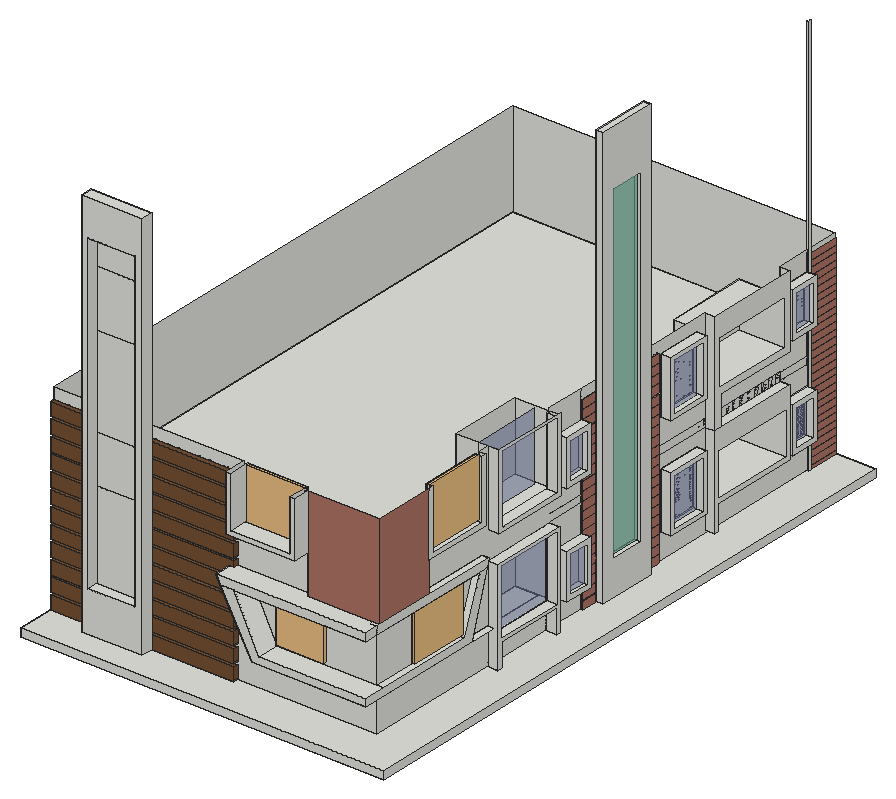
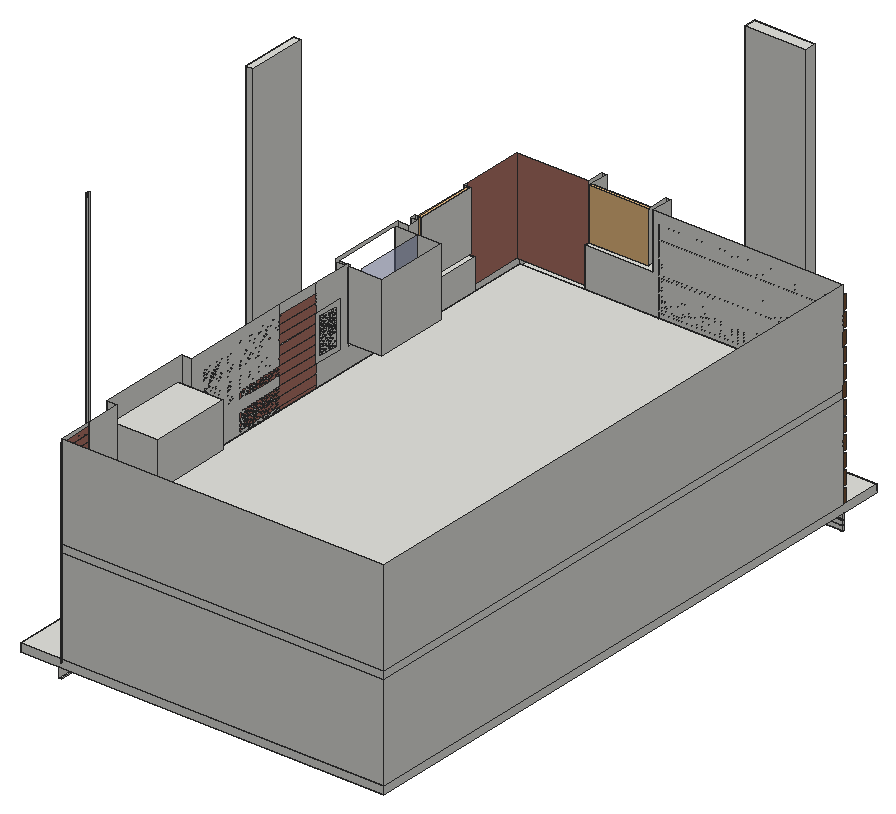
# SketchUp Ruby script. Lengths in inches.
U = 1.inch
M = Sketchup.active_model
def pt(a) = Geom::Point3d.new(a.map { |v| v * U })
def face(e, loops, mat)
  f = e.add_face(loops[0].map { |a| pt(a) })
  loops[1..].each { |l| e.add_face(l.map { |a| pt(a) }).erase! }
  f.material = f.back_material = mat if mat
  f
end
# faces: each face lists its corners as indices into pts; further lists are holes
def faces(e, pts, list, mat = nil) = list.each { |f| face(e, (f[0].is_a?(Array) ? f : [f]).map { |l| l.map { |i| pts[i] } }, mat) }
# xy, xz, yz: faces in a plane at the given z, y or x. An outline is a flat list of corners, or four numbers for a rectangle; further outlines are holes
def ring(l) = l.size == 4 ? [[l[0], l[1]], [l[2], l[1]], [l[2], l[3]], [l[0], l[3]]] : l.each_slice(2).to_a
def flat(e, list, mat, &to3) = list.each { |f| face(e, (f[0].is_a?(Array) ? f : [f]).map { |l| ring(l).map { |u, v| to3.(u, v) } }, mat) }
def xy(e, z, list, mat = nil) = flat(e, list, mat) { |x, y| [x, y, z] }
def xz(e, y, list, mat = nil) = flat(e, list, mat) { |x, z| [x, y, z] }
def yz(e, x, list, mat = nil) = flat(e, list, mat) { |y, z| [x, y, z] }
def lines(e, pts, list) = list.each { |a, b| e.add_line(pt(pts[a]), pt(pts[b])) }
# prism: a flat outline (further loops are holes) pulled along v
def prism(e, loops, v, mat = nil)
  f = face(e, loops, mat); d = Geom::Vector3d.new(v.map { |x| x * U })
  f.pushpull(f.normal.samedirection?(d) ? d.length : -d.length)
end
def box(e, o, s, mat = nil) = prism(e, [[o, [o[0] + s[0], o[1], o[2]], [o[0] + s[0], o[1] + s[1], o[2]], [o[0], o[1] + s[1], o[2]]]], [0, 0, s[2]], mat)
def at(x, y, z, deg = 0) = Geom::Transformation.translation(pt([x, y, z])) * Geom::Transformation.rotation(ORIGIN, Z_AXIS, deg.degrees)
def axes(o, x, y, z) = Geom::Transformation.new([*x, 0, *y, 0, *z, 0, *pt(o).to_a, 1])
def part(name) = M.definitions.add(name)
# library, detail: a bought-in or finely detailed component or shape, given as its bounding box
def library(name, o, s) = part(name).tap { |d| box(d.entities, o, s) }
def detail(e, o, s) = box(e.add_group.entities, o, s)
def put(e, d, t, mat = nil) = e.add_instance(d, t).tap { |i| i.material = mat if mat }
def group(e, t, mat = nil) = e.add_group.tap { |g| g.transformation = t; g.material = mat if mat }.entities
root = M.entities
M.materials.add("Artistic-Tile__Vetromarmi__Granada-Smoke-Glass-and-Stone-Wat").color = [172, 173, 170]
M.materials.add("MaterialE").color = [182, 131, 172]
M.materials["MaterialE"].alpha = 0.66
M.materials.add("MaterialF").color = [114, 188, 161]
M.materials["MaterialF"].alpha = 0.66
M.materials.add("[Sandstone]").color = [118, 81, 52]
M.materials.add("[Stone Flagstone Ashlar]").color = [175, 116, 102]
M.materials.add("[Terrazzo Tile Accent]").color = [224, 221, 217]
M.materials.add("[Translucent Glass Sky Reflection]").color = [126, 138, 183]
M.materials["[Translucent Glass Sky Reflection]"].alpha = 0.52
c1 = part("Group\#13")
box(c1.entities,[0,0,0],[1.1875,48.5625,8.8125])
c2 = part("Group\#12")
prism(c2.entities,[[[0,67.07,0],[0,0,0],[0,0,12.125],[0,67.07,12.125],[0,139.8125,12.125],[0,139.8125,0]]],[2.5,0,0])
c3 = part("Group\#11")
prism(c3.entities,[[[271.64,0,19.53],[271.64,0,2.36],[271.64,0,0],[0,0,0],[0,0,19.53]]],[0,-6.9375,0])
c4 = part("Artistic-Tile__Vetromarmi__Granada-Smoke-Glass-and-Stone-Wat")
xy(c4.entities,0,[[0,0,24,24]],"[Translucent Glass Sky Reflection]")
c5 = part("Group\#5")
xy(c5.entities,0,[[[0,0,66.75,83.5625],[5.83,5.83,60.92,77.73]],[5.83,5.83,60.92,77.73]])
xy(c5.entities,15.625,[[[0,0,66.75,83.5625],[5.83,5.83,60.92,77.73]]])
xz(c5.entities,0,[[0,0,66.75,15.625]])
xz(c5.entities,5.83,[[5.83,0,60.92,15.625]])
xz(c5.entities,77.73,[[5.83,0,60.92,15.625]])
xz(c5.entities,83.5625,[[0,0,66.75,15.625]])
yz(c5.entities,0,[[0,0,83.5625,15.625]])
yz(c5.entities,5.83,[[5.83,0,77.73,15.625]])
yz(c5.entities,60.92,[[5.83,0,77.73,15.625]])
yz(c5.entities,66.75,[[0,0,83.5625,15.625]])
c6 = part("Group\#6")
xy(c6.entities,0,[[[0,0,45,67.3125],[6.42,6.42,38.58,60.9]],[6.42,6.42,38.58,60.9]])
xy(c6.entities,14.3125,[[[0,0,45,67.3125],[6.42,6.42,38.58,60.9]]])
xz(c6.entities,0,[[0,0,45,14.3125]])
xz(c6.entities,6.42,[[6.42,0,38.58,14.3125]])
xz(c6.entities,60.9,[[6.42,0,38.58,14.3125]])
xz(c6.entities,67.3125,[[0,0,45,14.3125]])
yz(c6.entities,0,[[0,0,67.3125,14.3125]])
yz(c6.entities,6.42,[[6.42,0,60.9,14.3125]])
yz(c6.entities,38.58,[[6.42,0,60.9,14.3125]])
yz(c6.entities,45,[[0,0,67.3125,14.3125]])
c7 = part("glassE")
xy(c7.entities,0,[[0,0,37.99,0.79]],"MaterialE")
xy(c7.entities,38.27,[[0,0,37.99,0.79]],"MaterialE")
xz(c7.entities,0,[[0,0,37.99,38.27]],"MaterialF")
yz(c7.entities,0,[[0,0,0.79,38.27]],"MaterialE")
yz(c7.entities,37.99,[[0,0,0.79,38.27]],"MaterialE")
c8 = library("AS-120-mm\#2",[0,0,0],[88.21,4.72,72.97])
c9 = library("AS-120-mm",[0,0,0],[70.08,4.72,66.14])
c10 = library("AS-120-mm\#3",[0,0,0],[89.97,4.72,86.67])
c11 = library("AS-120-mm\#1",[0,0,0],[88.21,4.72,75.99])
xy(root,116.68,[[336.5625,87.66,386.78,90.47]])
xy(root,117.35,[[336.5625,87.66,386.78,90.47]])
xy(root,117.55,[[750.91,87.66,816.1875,87.66,816.1875,140.66,814.625,140.66,814.625,90.47,750.91,90.47]])
xy(root,117.93,[[750.91,87.66,750.91,90.47,814.625,90.47,814.625,140.66,816.1875,140.66,816.1875,87.66]])
xy(root,118.17,[[547.16,87.66,593.34,90.47]])
xy(root,118.57,[[547.16,87.66,593.34,90.47]])
xy(root,122.17,[[814.625,263.05,816.1875,305.04]])
xy(root,122.8125,[[814.625,263.05,816.1875,305.04]])
xy(root,123.57,[[336.5625,87.66,386.78,90.47]])
xy(root,124.47,[[336.5625,87.66,386.78,90.47]])
xy(root,125.05,[[547.16,87.66,593.34,90.47]])
xy(root,125.11,[[750.91,87.66,816.1875,87.66,816.1875,140.66,814.625,140.66,814.625,90.47,750.91,90.47]])
xy(root,125.12,[[814.625,423.33,816.875,495.84]])
xy(root,125.29,[[814.625,599,817.6875,719.91]])
xy(root,125.4,[[547.16,87.66,593.34,90.47],[750.91,87.66,750.91,90.47,814.625,90.47,814.625,140.66,816.1875,140.66,816.1875,87.66]])
xy(root,126.33,[[814.625,423.33,816.875,495.84],[814.625,599,817.6875,939.04]])
xy(root,130.29,[[814.625,263.05,816.1875,305.04]])
xy(root,130.7,[[336.5625,87.66,386.78,90.47]])
xy(root,131.62,[[336.5625,87.66,386.78,90.47],[386.78,87.66,547.16,90.47],[547.16,87.66,593.34,90.47],[593.34,87.66,750.91,90.47],[750.91,87.66,797.1,90.47],
  [797.1,87.66,797.1,90.47,814.625,90.47,814.625,140.66,816.1875,140.66,816.1875,87.66],[814.625,140.66,816.1875,305.04]])
xy(root,140.0625,[[336.5625,87.66,816.1875,87.66,816.1875,423.33,816.875,423.33,816.875,495.84,814.625,495.84,814.625,599,817.6875,599,817.6875,939.04,336.5625,939.04]])
xy(root,152.0625,[[396.82,65.66,486.94,83.54],[336.5625,90.47,336.5625,939.04,814.625,939.04,814.625,409.52,763.75,409.52,763.75,295.05,814.625,295.05,814.625,90.47],[799.03,295.05,814.625,409.52],[814.625,295.05,830.625,302.34],[814.625,403.375,830.625,409.52],
  [814.625,886.91,817.0625,890.48]])
xy(root,152.39,[[817.125,492.91,827.875,580.72]])
xy(root,155.57,[[814.625,697.51,828.9375,704.04]])
xy(root,187.1875,[[814.625,302.34,830.625,403.375]])
xy(root,190.375,[[763.75,295.05,799.03,300.49],[763.75,300.49,799.03,409.52]])
xy(root,191.375,[[799.03,295.05,814.625,300.49],[799.03,300.49,814.625,409.52],[814.625,300.49,830.625,404.56]])
xy(root,193.01,[[814.625,704.04,828.9375,837.09]])
xy(root,199.04,[[739.5625,703.54,828.9375,831.06]])
xy(root,204.33,[[817.6875,510.98,827.875,562.65]])
xy(root,206.05,[[655.6,57.85,824.98,90.47],[814.625,90.47,824.98,252.35],[814.625,252.35,824.98,256.15],[814.625,256.15,824.98,295.05]])
xy(root,212.49,[[406.93,65.66,476.45,81.97]])
xy(root,216.42,[[666.1875,57.85,824.98,90.47],[814.625,90.47,824.98,241.1]])
xy(root,262.84,[[739.5625,703.54,828.9375,831.06]])
xy(root,288.85,[[763.75,300.49,763.75,409.52,814.625,409.52,814.625,404.56,830.625,404.56,830.625,300.49]])
xy(root,292.125,[[608.76,57.85,628.31,57.85,628.31,90.47,814.625,90.47,814.625,267.45,824.98,267.45,824.98,280.55,814.625,280.55,814.625,939.04,336.5625,939.04,336.5625,90.47,608.76,90.47],[608.2,57.85,608.76,90.47],[628.31,57.85,628.31,90.47,814.625,90.47,814.625,77.97,824.98,77.97,824.98,57.85],[814.625,77.97,824.98,267.45],[814.625,295.05,830.625,409.52],
  [814.625,708.96,828.9375,837.09]])
xy(root,304.125,[[602.42,57.85,824.98,57.85,824.98,77.97,814.625,77.97,814.625,83.16,718.625,83.16,718.625,90.47,602.42,90.47],[814.625,77.97,824.98,83.16],[814.625,174.47,824.98,284.49]])
xy(root,333.5625,[[814.625,295.05,831,409.52]])
xy(root,336.72,[[814.625,708.96,828.9375,837.09]])
xy(root,339.375,[[763.75,300.49,814.625,409.52],[814.625,300.49,831,404.56]])
xy(root,341.89,[[406.93,81.97,476.45,82.04]])
xy(root,345.47,[[761,706.26,828.9375,828.35]])
xy(root,349.61,[[814.625,174.47,824.98,278.47]])
xy(root,356.41,[[814.625,181.28,824.98,271.67]])
xy(root,362.03,[[616.81,57.85,718.625,90.47]])
xy(root,368.84,[[623.61,57.85,711.82,90.47]])
xy(root,412.625,[[761,706.26,828.9375,828.35]])
xy(root,412.83,[[406.93,82.04,476.45,82.1]])
xy(root,548.48,[[406.93,82.04,476.45,82.1]])
xy(root,633.26,[[406.93,82.04,476.45,82.1]])
xy(root,678.16,[[406.93,65.66,476.45,82.1]])
xy(root,694.59,[[817.6875,510.98,827.875,562.65]])
xy(root,731.15,[[396.82,65.66,486.94,83.54]])
xy(root,777,[[817.125,492.91,827.875,580.72]])
xz(root,57.85,[[655.16,205.82,655.6,206.05,824.98,206.05,824.98,216.42,666.1875,216.42,628.31,292.125,608.76,292.125,608.33,291.89],[608.2,292.125,824.98,292.125,824.98,304.125,602.42,304.125],[616.81,362.03,718.625,362.03,718.625,444.1875,711.82,444.1875,711.82,368.84,623.61,368.84,623.61,444.1875,616.81,444.1875]])
xz(root,65.66,[[[396.82,152.0625,486.94,731.15],[406.93,212.49,476.45,678.16]]])
xz(root,81.97,[[406.93,212.49,476.45,341.89]])
xz(root,82.04,[[406.93,341.89,476.45,412.83],[406.93,548.48,476.45,633.26]])
xz(root,82.1,[[406.93,412.83,476.45,548.48],[406.93,633.26,476.45,678.16]])
xz(root,83.16,[[718.625,304.125,824.98,444.1875]],"[Stone Flagstone Ashlar]")
xz(root,83.54,[[396.82,152.0625,486.94,731.15]])
xz(root,87.66,[[336.5625,117.35,386.78,123.57],[750.91,117.93,816.1875,125.11],[547.16,118.57,593.34,125.05],[336.5625,124.47,386.78,130.7],[547.16,125.4,593.34,131.62],
  [750.91,125.4,816.1875,131.62],[336.5625,131.62,816.1875,140.0625]],"[Terrazzo Tile Accent]")
xz(root,90.47,[[336.5625,116.68,386.78,117.35],[336.5625,117.35,386.78,123.57],[750.91,117.55,814.625,117.93],[750.91,117.93,814.625,125.11],[547.16,118.17,593.34,118.57],
  [336.5625,123.57,386.78,124.47],[336.5625,124.47,386.78,130.7],[547.16,125.05,593.34,125.4],[750.91,125.11,814.625,125.4],[547.16,125.4,593.34,131.62],
  [750.91,125.4,814.625,131.62],[336.5625,130.7,386.78,131.62],[336.5625,152.0625,814.625,152.0625,814.625,206.05,655.6,206.05,655.16,205.82,608.33,291.89,608.76,292.125,336.5625,292.125],[666.1875,216.42,814.625,216.42,814.625,292.125,628.31,292.125],[336.5625,304.125,718.625,304.125,718.625,362.03,616.81,362.03,616.81,444.1875,336.5625,444.1875],
  [623.61,368.84,711.82,444.1875]])
xz(root,140.66,[[814.625,117.93,816.1875,125.11],[814.625,125.4,816.1875,131.62]])
xz(root,174.47,[[814.625,304.125,824.98,349.61]])
xz(root,181.28,[[814.625,356.41,824.98,444.1875]])
xz(root,263.05,[[814.625,122.8125,816.1875,130.29]])
xz(root,271.67,[[814.625,356.41,824.98,444.1875]])
xz(root,278.47,[[814.625,349.61,824.98,444.1875]])
xz(root,295.05,[[763.75,152.0625,799.03,190.375],[814.625,152.0625,830.625,292.125],[814.625,333.5625,831,444.1875]])
xz(root,300.49,[[763.75,190.375,763.75,288.85,830.625,288.85,830.625,191.375,799.03,191.375,799.03,190.375],[763.75,339.375,831,440.43]])
xz(root,302.34,[[814.625,152.0625,830.625,187.1875]])
xz(root,305.04,[[814.625,122.17,816.1875,122.8125],[814.625,130.29,816.1875,131.62]])
xz(root,403.375,[[814.625,152.0625,830.625,187.1875]])
xz(root,404.56,[[814.625,191.375,830.625,288.85],[814.625,339.375,831,440.43]])
xz(root,409.52,[[763.75,152.0625,799.03,190.375],[814.625,152.0625,830.625,288.85],[763.75,190.375,763.75,288.85,814.625,288.85,814.625,191.375,799.03,191.375,799.03,190.375],[763.75,288.85,814.625,292.125],[814.625,288.85,830.625,292.125],
  [814.625,333.5625,831,440.43],[763.75,339.375,814.625,440.43]])
xz(root,423.33,[[814.625,125.12,816.1875,126.33],[816.1875,126.33,816.875,140.0625]])
xz(root,492.91,[[817.125,152.39,827.875,777]])
xz(root,495.84,[[814.625,126.33,816.875,140.0625]])
xz(root,510.98,[[817.6875,204.33,827.875,694.59]])
xz(root,562.65,[[817.6875,204.33,827.875,694.59]])
xz(root,580.72,[[817.125,152.39,827.875,777]])
xz(root,599,[[814.625,126.33,817.6875,140.0625]])
xz(root,697.51,[[814.625,155.57,828.9375,292.125],[814.625,292.125,828.9375,443.8125]])
xz(root,703.54,[[739.5625,199.04,828.9375,262.84]])
xz(root,704.04,[[814.625,155.57,828.9375,193.01]])
xz(root,706.26,[[761,345.47,828.9375,412.625]])
xz(root,708.96,[[814.625,292.125,828.9375,336.72]])
xz(root,828.35,[[761,345.47,828.9375,412.625]])
xz(root,831.06,[[739.5625,199.04,828.9375,262.84]])
xz(root,837.09,[[814.625,193.01,828.9375,292.125],[814.625,336.72,828.9375,444.1875]])
xz(root,886.91,[[814.625,152.0625,817.0625,748.3125]])
xz(root,890.48,[[814.625,152.0625,814.625,742.93,815.8125,742.93,815.8125,748.3125,817.0625,748.3125,817.0625,152.0625]])
xz(root,939.04,[[336.5625,152.0625,814.625,292.125],[336.5625,304.125,814.625,444.1875]])
yz(root,336.5625,[[87.66,117.35,90.47,123.57],[87.66,124.47,90.47,130.7],[87.66,131.62,90.47,140.0625],[90.47,152.0625,939.04,292.125],[90.47,304.125,939.04,444.1875]])
yz(root,386.78,[[87.66,117.35,90.47,123.57],[87.66,124.47,90.47,130.7]])
yz(root,396.82,[[65.66,152.0625,83.54,731.15]])
yz(root,406.93,[[65.66,212.49,81.97,212.49,81.97,341.89,82.04,341.89,82.04,412.83,82.1,412.83,82.1,548.48,82.04,548.48,82.04,633.26,82.1,633.26,82.1,678.16,65.66,678.16]])
yz(root,476.45,[[65.66,212.49,65.66,678.16,82.1,678.16,82.1,633.26,82.04,633.26,82.04,548.48,82.1,548.48,82.1,412.83,82.04,412.83,82.04,341.89,81.97,341.89,81.97,212.49]])
yz(root,486.94,[[65.66,152.0625,83.54,731.15]])
yz(root,547.16,[[87.66,118.57,90.47,125.05],[87.66,125.4,90.47,131.62]])
yz(root,593.34,[[87.66,118.57,90.47,125.05],[87.66,125.4,90.47,131.62]])
yz(root,616.81,[[57.85,362.03,90.47,444.1875]])
yz(root,623.61,[[57.85,368.84,90.47,444.1875]])
yz(root,711.82,[[57.85,368.84,90.47,444.1875]])
yz(root,718.625,[[83.16,304.125,90.47,362.03],[57.85,362.03,83.16,444.1875]])
yz(root,739.5625,[[703.54,199.04,831.06,262.84]])
yz(root,750.91,[[87.66,117.93,90.47,125.11],[87.66,125.4,90.47,131.62]])
yz(root,761,[[706.26,345.47,828.35,412.625]])
yz(root,763.75,[[295.05,152.0625,409.52,190.375],[300.49,190.375,409.52,288.85],[300.49,339.375,409.52,440.43]])
yz(root,799.03,[[295.05,152.0625,409.52,190.375],[295.05,190.375,300.49,191.375],[300.49,190.375,409.52,191.375]])
yz(root,814.625,[[90.47,117.93,140.66,125.11],[263.05,122.17,305.04,122.8125],[423.33,125.12,495.84,126.33],[599,125.29,939.04,126.33],[90.47,125.4,140.66,131.62],
  [263.05,130.29,305.04,131.62],[90.47,152.0625,295.05,206.05],[295.05,152.0625,302.34,152.0625,302.34,187.1875,403.375,187.1875,403.375,152.0625,409.52,152.0625,409.52,191.375,295.05,191.375],[302.34,152.0625,403.375,187.1875],[409.52,152.0625,468.48,292.125],
  [468.48,152.0625,535.54,292.125],[535.54,152.0625,886.91,152.0625,886.91,292.125,837.09,292.125,837.09,193.01,704.04,193.01,704.04,155.57,697.51,155.57,697.51,292.125,535.54,292.125],[890.48,152.0625,939.04,292.125],[404.56,191.375,409.52,288.85],[252.35,206.05,295.05,206.05,295.05,292.125,280.55,292.125],
  [90.47,216.42,241.1,216.42,267.45,292.125,90.47,292.125],[280.55,292.125,468.48,292.125,468.48,444.1875,409.52,444.1875,409.52,333.5625,295.05,333.5625,295.05,444.1875,278.47,444.1875,278.47,349.61,174.47,349.61,174.47,304.125,284.49,304.125],[468.48,292.125,535.54,304.125],[535.54,292.125,697.51,304.125],[708.96,292.125,837.09,304.125],
  [886.91,292.125,890.48,304.125],[468.48,304.125,535.54,444.1875],[535.54,304.125,697.51,444.1875],[708.96,304.125,886.91,304.125,886.91,444.1875,837.09,444.1875,837.09,336.72,708.96,336.72],[886.91,304.125,890.48,444.1875],
  [890.48,304.125,939.04,444.1875],[404.56,339.375,409.52,440.43],[181.28,356.41,271.67,444.1875]])
yz(root,816.1875,[[87.66,117.93,140.66,125.11],[263.05,122.8125,305.04,130.29],[87.66,125.4,140.66,131.62],[87.66,131.62,305.04,140.0625]],"[Terrazzo Tile Accent]")
yz(root,816.875,[[423.33,126.33,495.84,140.0625]],"[Terrazzo Tile Accent]")
yz(root,817.0625,[[886.91,152.0625,890.48,748.3125]])
yz(root,817.125,[[492.91,152.39,580.72,777]])
yz(root,817.6875,[[510.98,204.33,562.65,694.59]])
yz(root,817.6875,[[599,126.33,939.04,140.0625]],"[Terrazzo Tile Accent]")
yz(root,824.98,[[57.85,206.05,252.35,206.05,280.55,292.125,267.45,292.125,241.1,216.42,57.85,216.42],[57.85,292.125,77.97,304.125],[77.97,292.125,280.55,292.125,284.49,304.125,77.97,304.125],[174.47,349.61,278.47,349.61,278.47,444.1875,271.67,444.1875,271.67,356.41,181.28,356.41,181.28,444.1875,174.47,444.1875]])
yz(root,824.98,[[83.16,304.125,174.47,444.1875]],"[Stone Flagstone Ashlar]")
yz(root,827.875,[[[492.91,152.39,580.72,777],[510.98,204.33,562.65,694.59]]])
yz(root,828.9375,[[[697.51,155.57,704.04,155.57,704.04,193.01,837.09,193.01,837.09,292.125,697.51,292.125],[703.54,199.04,831.06,262.84]],[[697.51,292.125,708.96,292.125,708.96,336.72,837.09,336.72,837.09,444.1875,697.51,444.1875],[706.26,345.47,828.35,412.625]]])
yz(root,830.625,[[[295.05,152.0625,302.34,152.0625,302.34,187.1875,403.375,187.1875,403.375,152.0625,409.52,152.0625,409.52,292.125,295.05,292.125],[300.49,191.375,404.56,288.85]]])
yz(root,831,[[[295.05,333.5625,409.52,444.1875],[300.49,339.375,404.56,440.43]]])
p = [[608.33,90.47,291.89],[655.16,90.47,205.82],[655.16,57.85,205.82],[608.33,57.85,291.89],[608.33,77.97,291.89],[655.6,90.47,206.05],
  [655.6,57.85,206.05],[814.625,252.35,206.05],[814.625,280.55,292.125],[824.98,280.55,292.125],[824.98,252.35,206.05],[666.1875,90.47,216.42],
  [628.31,90.47,292.125],[628.31,57.85,292.125],[666.1875,57.85,216.42],[814.625,267.45,292.125],[814.625,241.1,216.42],[824.98,241.1,216.42],
  [824.98,267.45,292.125],[608.76,57.85,292.125],[608.76,77.97,292.125],[608.76,90.47,292.125],[602.42,90.47,304.125],[608.2,90.47,292.125],
  [608.2,57.85,292.125],[602.42,57.85,304.125],[814.625,284.49,304.125],[824.98,284.49,304.125],[814.625,409.52,304.125],[814.625,468.48,304.125],
  [814.625,295.05,157],[799.03,295.05,157],[814.625,300.49,155.9375],[799.03,295.05,152.0625]]
faces(root,p,[[0,1,2,3,4],[5,6,2,1],[7,8,9,10],[11,12,13,14],[15,16,17,18],[19,20,4,3],[20,21,0,4],[22,23,24,25],
  [8,26,27,9]])
lines(root,p,[[28,29],[30,31],[32,33]])
g1 = group(root,at(336.5625,690.47,140.0625))
box(g1,[0,-662.625,0],[538.8125,911.1875,12])
put(root,c1,at(814.625,890.48,146.75),"[Stone Flagstone Ashlar]")
put(root,c2,at(814.625,468.48,150.48),"[Stone Flagstone Ashlar]")
put(root,c3,at(336.5625,90.47,152.12),"[Sandstone]")
put(root,c1,at(814.625,890.48,156.75),"[Stone Flagstone Ashlar]")
put(root,c2,at(814.625,468.48,164.29),"[Stone Flagstone Ashlar]")
put(root,c1,at(814.625,890.48,166.75),"[Stone Flagstone Ashlar]")
put(root,c3,at(336.5625,90.47,175.43),"[Sandstone]")
put(root,c1,at(814.625,890.48,176.75),"[Stone Flagstone Ashlar]")
put(root,c2,at(814.625,468.48,177.71),"[Stone Flagstone Ashlar]")
g2 = group(root,at(814.625,423.48,185.41))
xy(g2,0,[[0,0,14.3125,45]])
xy(g2,6.42,[[0,6.42,14.3125,38.58]])
xy(g2,60.9,[[0,6.42,14.3125,38.58]])
xy(g2,67.3125,[[0,0,14.3125,45]])
xz(g2,0,[[0,0,14.3125,67.3125]])
xz(g2,6.42,[[0,6.42,14.3125,60.9]])
xz(g2,38.58,[[0,6.42,14.3125,60.9]])
xz(g2,45,[[0,0,14.3125,67.3125]])
yz(g2,0,[[[0,0,45,67.3125],[6.42,6.42,38.58,60.9]],[6.42,6.42,38.58,60.9]])
yz(g2,14.3125,[[[0,0,45,67.3125],[6.42,6.42,38.58,60.9]]])
put(root,c4,axes([813.12,404.56,287.11],[0,-4.33639,0],[0,0,-4.22736],[1,0,0]))
put(root,c1,at(814.625,890.48,186.75),"[Stone Flagstone Ashlar]")
put(root,c5,axes([814.625,615.15,189.68],[0,1,0],[0,0,1],[1,0,0]))
put(root,c2,at(814.625,468.48,190.89),"[Stone Flagstone Ashlar]")
put(root,c4,axes([824.82,461.8125,246.31],[0,-1.33,0],[0,0,-2.26992],[1,0,0]))
put(root,c6,axes([814.625,841.91,196.54],[0,1,0],[0,0,1],[1,0,0]))
put(root,c1,at(814.625,890.48,196.75),"[Stone Flagstone Ashlar]")
put(root,c4,axes([822.4375,672.37,270.09],[0,-2.1413,0],[0,0,-3.0449],[1,0,0]))
put(root,c3,at(336.5625,90.47,198.74),"[Sandstone]")
put(root,c4,axes([820,880.25,257.43],[0,-1.33,0],[0,0,-2.26992],[1,0,0]))
put(root,c2,at(814.625,468.48,204.08),"[Stone Flagstone Ashlar]")
put(root,c7,axes([822.78,562.65,205.53],[0,-1.36,0],[1,0,0],[0,0,12.78]))
put(root,c1,at(814.625,890.48,206.75),"[Stone Flagstone Ashlar]")
put(root,c1,at(814.625,890.48,216.75),"[Stone Flagstone Ashlar]")
put(root,c2,at(814.625,468.48,217.27),"[Stone Flagstone Ashlar]")
put(root,c8,at(815.625,241.9,219.15,-90))
put(root,c9,at(668.92,85.75,220.625))
put(root,c3,at(336.5625,90.47,222.05),"[Sandstone]")
put(root,c1,at(814.625,890.48,226.75),"[Stone Flagstone Ashlar]")
put(root,c2,at(814.625,468.48,230.46),"[Stone Flagstone Ashlar]")
put(root,c1,at(814.625,890.48,236.875),"[Stone Flagstone Ashlar]")
put(root,c2,at(814.625,468.48,243.64),"[Stone Flagstone Ashlar]")
put(root,c3,at(336.5625,90.47,245.37),"[Sandstone]")
put(root,c1,at(814.625,890.48,247),"[Stone Flagstone Ashlar]")
put(root,c2,at(814.625,468.48,256.83),"[Stone Flagstone Ashlar]")
put(root,c1,at(814.625,890.48,257.125),"[Stone Flagstone Ashlar]")
put(root,c1,at(814.625,890.48,267.25),"[Stone Flagstone Ashlar]")
put(root,c3,at(336.5625,90.47,268.68),"[Sandstone]")
put(root,c2,at(814.625,468.48,270.02),"[Stone Flagstone Ashlar]")
put(root,c1,at(814.625,890.48,277.375),"[Stone Flagstone Ashlar]")
put(root,c2,at(814.625,468.48,283.21),"[Stone Flagstone Ashlar]")
put(root,c1,at(814.625,890.48,287.5),"[Stone Flagstone Ashlar]")
put(root,c3,at(336.5625,90.47,291.99),"[Sandstone]")
g3 = group(root,at(336.5625,690.47,292.125))
box(g3,[0,-600,0],[478.0625,848.5625,12])
put(root,c2,at(814.625,468.48,296.39),"[Stone Flagstone Ashlar]")
put(root,c1,at(814.625,890.48,297.625),"[Stone Flagstone Ashlar]")
put(root,c1,at(814.625,890.48,307.75),"[Stone Flagstone Ashlar]")
put(root,c2,at(814.625,468.48,309.58),"[Stone Flagstone Ashlar]")
put(root,c3,at(336.5625,90.47,315.3),"[Sandstone]")
put(root,c1,at(814.625,890.48,317.875),"[Stone Flagstone Ashlar]")
put(root,c2,at(814.625,468.48,323.14),"[Stone Flagstone Ashlar]")
put(root,c1,at(814.625,890.48,328),"[Stone Flagstone Ashlar]")
g4 = group(root,at(814.625,423.48,336.41))
xy(g4,0,[[0,0,14.3125,45]])
xy(g4,6.42,[[0,6.42,14.3125,38.58]])
xy(g4,60.9,[[0,6.42,14.3125,38.58]])
xy(g4,67.3125,[[0,0,14.3125,45]])
xz(g4,0,[[0,0,14.3125,67.3125]])
xz(g4,6.42,[[0,6.42,14.3125,60.9]])
xz(g4,38.58,[[0,6.42,14.3125,60.9]])
xz(g4,45,[[0,0,14.3125,67.3125]])
yz(g4,0,[[[0,0,45,67.3125],[6.42,6.42,38.58,60.9]],[6.42,6.42,38.58,60.9]])
yz(g4,14.3125,[[[0,0,45,67.3125],[6.42,6.42,38.58,60.9]]])
put(root,c2,at(814.625,468.48,336.71),"[Stone Flagstone Ashlar]")
put(root,c1,at(814.625,890.48,338.125),"[Stone Flagstone Ashlar]")
put(root,c3,at(336.5625,90.47,338.62),"[Sandstone]")
put(root,c4,axes([797.375,404.56,440.43],[0,-4.33639,0],[0,0,-4.22736],[1,0,0]))
put(root,c5,axes([814.625,615.15,342.68],[0,1,0],[0,0,1],[1,0,0]))
put(root,c4,axes([822.8125,462.06,397.31],[0,-1.33,0],[0,0,-2.26992],[1,0,0]))
put(root,c4,axes([822.4375,672.37,420.27],[0,-2.1413,0],[0,0,-3.0449],[1,0,0]))
put(root,c1,at(814.625,890.48,348.25),"[Stone Flagstone Ashlar]")
put(root,c6,axes([814.625,841.91,348.47],[0,1,0],[0,0,1],[1,0,0]))
put(root,c2,at(814.625,468.48,350.27),"[Stone Flagstone Ashlar]")
put(root,c4,axes([824.25,880.25,409.37],[0,-1.33,0],[0,0,-2.26992],[1,0,0]))
put(root,c10,at(815.48,271.67,357.75,-90))
put(root,c1,at(814.625,890.48,358.375),"[Stone Flagstone Ashlar]")
put(root,c3,at(336.5625,90.47,361.93),"[Sandstone]")
put(root,c2,at(814.625,468.48,363.83),"[Stone Flagstone Ashlar]")
put(root,c11,at(623.61,85.95,368.2))
put(root,c1,at(814.625,890.48,368.5),"[Stone Flagstone Ashlar]")
put(root,c2,at(814.625,468.48,377.39),"[Stone Flagstone Ashlar]")
put(root,c1,at(814.625,890.48,378.625),"[Stone Flagstone Ashlar]")
put(root,c3,at(336.5625,90.47,385.24),"[Sandstone]")
put(root,c1,at(814.625,890.48,388.75),"[Stone Flagstone Ashlar]")
put(root,c2,at(814.625,468.48,390.96),"[Stone Flagstone Ashlar]")
put(root,c1,at(814.625,890.48,398.875),"[Stone Flagstone Ashlar]")
put(root,c2,at(814.625,468.48,404.52),"[Stone Flagstone Ashlar]")
put(root,c3,at(336.5625,90.47,408.55),"[Sandstone]")
put(root,c1,at(814.625,890.48,409),"[Stone Flagstone Ashlar]")
put(root,c2,at(814.625,468.48,418.08),"[Stone Flagstone Ashlar]")
put(root,c1,at(814.625,890.48,419.125),"[Stone Flagstone Ashlar]")
put(root,c1,at(814.625,890.48,429.25),"[Stone Flagstone Ashlar]")
